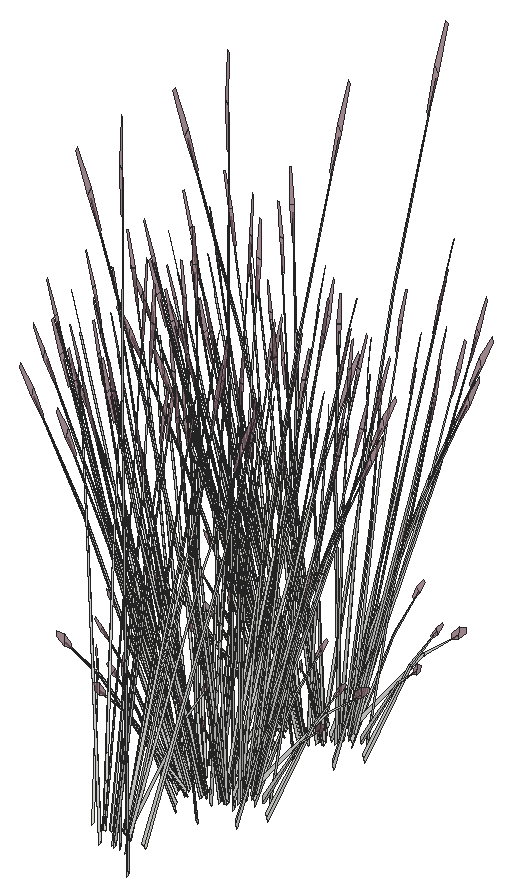
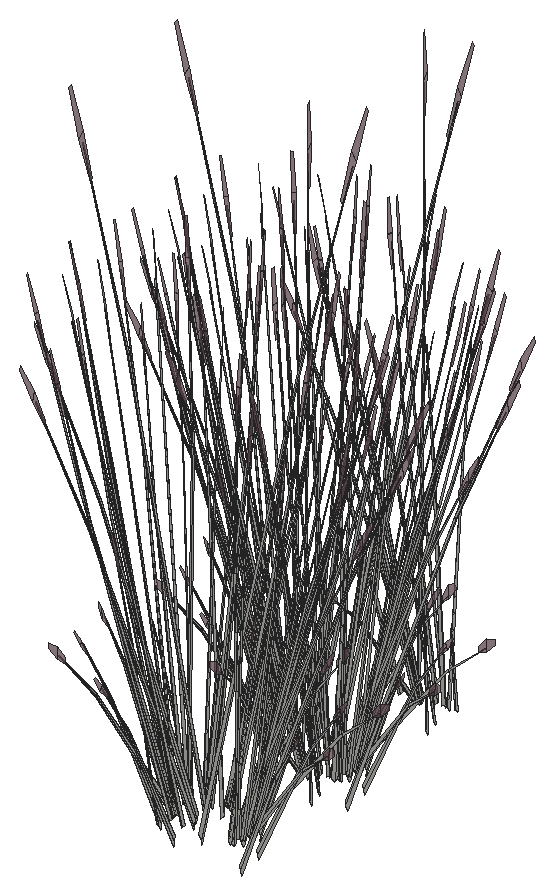
# SketchUp Ruby script. Lengths in inches.
U = 1.inch
M = Sketchup.active_model
def pt(a) = Geom::Point3d.new(a.map { |v| v * U })
def face(e, loops, mat)
  f = e.add_face(loops[0].map { |a| pt(a) })
  loops[1..].each { |l| e.add_face(l.map { |a| pt(a) }).erase! }
  f.material = f.back_material = mat if mat
  f
end
# faces: each face lists its corners as indices into pts; further lists are holes
def faces(e, pts, list, mat = nil) = list.each { |f| face(e, (f[0].is_a?(Array) ? f : [f]).map { |l| l.map { |i| pts[i] } }, mat) }
# xy, xz, yz: faces in a plane at the given z, y or x. An outline is a flat list of corners, or four numbers for a rectangle; further outlines are holes
def ring(l) = l.size == 4 ? [[l[0], l[1]], [l[2], l[1]], [l[2], l[3]], [l[0], l[3]]] : l.each_slice(2).to_a
def flat(e, list, mat, &to3) = list.each { |f| face(e, (f[0].is_a?(Array) ? f : [f]).map { |l| ring(l).map { |u, v| to3.(u, v) } }, mat) }
def xy(e, z, list, mat = nil) = flat(e, list, mat) { |x, y| [x, y, z] }
def xz(e, y, list, mat = nil) = flat(e, list, mat) { |x, z| [x, y, z] }
def yz(e, x, list, mat = nil) = flat(e, list, mat) { |y, z| [x, y, z] }
def lines(e, pts, list) = list.each { |a, b| e.add_line(pt(pts[a]), pt(pts[b])) }
# prism: a flat outline (further loops are holes) pulled along v
def prism(e, loops, v, mat = nil)
  f = face(e, loops, mat); d = Geom::Vector3d.new(v.map { |x| x * U })
  f.pushpull(f.normal.samedirection?(d) ? d.length : -d.length)
end
def box(e, o, s, mat = nil) = prism(e, [[o, [o[0] + s[0], o[1], o[2]], [o[0] + s[0], o[1] + s[1], o[2]], [o[0], o[1] + s[1], o[2]]]], [0, 0, s[2]], mat)
def at(x, y, z, deg = 0) = Geom::Transformation.translation(pt([x, y, z])) * Geom::Transformation.rotation(ORIGIN, Z_AXIS, deg.degrees)
def axes(o, x, y, z) = Geom::Transformation.new([*x, 0, *y, 0, *z, 0, *pt(o).to_a, 1])
def part(name) = M.definitions.add(name)
# library, detail: a bought-in or finely detailed component or shape, given as its bounding box
def library(name, o, s) = part(name).tap { |d| box(d.entities, o, s) }
def detail(e, o, s) = box(e.add_group.entities, o, s)
def put(e, d, t, mat = nil) = e.add_instance(d, t).tap { |i| i.material = mat if mat }
def group(e, t, mat = nil) = e.add_group.tap { |g| g.transformation = t; g.material = mat if mat }.entities
root = M.entities
M.materials.add("LightPink_Translucent").color = [144, 107, 117]
M.materials["LightPink_Translucent"].alpha = 0.75
c1 = part("blade")
p = [[2.15,0.21,22],[0,0.17,0],[0.09,0.45,0],[2.18,0.31,22],[2.29,0.31,22],[0.38,0.45,0],
  [2.48,0.24,33],[2.49,0.24,33],[2.48,0.22,33]]
faces(c1.entities,p,[[0,1,2,3],[4,5,2,3],[6,3,4,7],[8,0,3,6]])
c2 = part("seeds")
p = [[0.3,-0.1,1.38],[-0.01,-0.03,1.59],[-0.01,-0.03,0.03],[0.14,-0.07,-0.07],[0.29,-0.03,3],[0.15,0.01,3.11]]
faces(c2.entities,p,[[0,1,2,3],[1,0,4,5]],"LightPink_Translucent")
c3 = part("blade with seeds")
put(c3.entities,c1,at(0,0,0))
put(c3.entities,c2,axes([2.4,0.25,30.99],[1.5799,-0.05474,1.17369],[-0.12525,1.92788,0.29478],[-0.07173,-0.02425,1.56792]))
put(root,c3,axes([334.74,276.7,50.51],[-0.01379,-0.36791,1.24828],[0.62424,0.09537,0.52853],[-0.14764,0.20132,1.17828]))
put(root,c3,axes([334.79,278.125,52.14],[0.49824,-0.09289,-0.45151],[0.08716,0.35177,-0.34973],[0.13382,0.10081,0.86392]))
put(root,c3,axes([332.16,277.37,51.43],[0.09401,-0.13431,1.51428],[0.3944,0.27795,0.12244],[-0.17792,0.17323,0.64734]))
put(root,c3,axes([332.27,278.13,52],[-0.34164,0.20573,-0.31292],[-0.3234,-0.23491,0.40398],[-0.04921,0.11936,0.77298]))
put(root,c3,axes([331.09,278.07,52.17],[-0.01255,0.07733,1.54581],[0.35618,0.269,-0.24447],[-0.09325,0.12721,0.12397]))
put(root,c3,axes([333.25,278.3,52.45],[0.49409,-0.18193,-0.10745],[0.24281,0.32289,-0.59638],[0.06519,0.13607,0.90619]))
put(root,c3,axes([332.48,278.93,50.44],[-0.01307,-0.23234,1.01491],[0.32652,0.16572,0.74569],[-0.06422,0.11074,0.22354]))
put(root,c3,axes([332.61,278.03,52.42],[0.36145,0.26255,-0.50118],[-0.38183,0.22994,-0.3882],[-0.055,0.1334,0.95895]))
put(root,c3,axes([333.68,278.29,52.14],[0.49634,0.09796,-0.45151],[-0.17013,0.33585,-0.34973],[0.04551,0.13522,0.86392]))
put(root,c3,axes([333.96,277.59,51.43],[-0.11542,-0.12546,1.51428],[0.53333,-0.10562,0.12244],[0.12054,0.19696,0.64734]))
put(root,c3,axes([333.45,278.49,52],[-0.15222,0.30049,-0.31292],[-0.44409,-0.08764,0.40398],[0.04072,0.12098,0.77298]))
put(root,c3,axes([332.49,277.91,52.72],[-0.01314,0.36145,-0.69681],[-0.55324,-0.02428,0.08409],[-0.05838,0.15313,0.9857]))
put(root,c3,axes([333.02,277.66,51.43],[-0.01236,-0.14998,1.51428],[0.53562,0.09949,0.12244],[-0.03313,0.21373,0.64734]))
put(root,c3,axes([333.5,278.22,52.4],[0.24099,0.31773,-0.62776],[-0.49607,0.17707,0.07576],[0.05635,0.15352,0.88802]))
put(root,c3,axes([332.69,284.9375,51.43],[0.11542,0.12546,1.51428],[-0.53333,0.10562,0.12244],[-0.12054,-0.19696,0.64734]))
put(root,c3,axes([333.14,279.03,52.17],[0.064,0.06292,1.54581],[0.51651,0.02472,-0.24447],[0.05194,0.13877,0.12397]))
put(root,c3,axes([333.57,284.11,52.17],[-0.07723,-0.05479,1.54581],[-0.51538,0.03473,-0.24447],[-0.08225,-0.13104,0.12397]))
put(root,c3,axes([334.11,285.03,52.4],[-0.24099,-0.31773,-0.62776],[0.49607,-0.17707,0.07576],[-0.05635,-0.15352,0.88802]))
put(root,c3,axes([332.31,278.42,50.97],[0.01109,-0.20172,1.3638],[0.49896,0.10655,0.18846],[-0.04323,0.21498,0.64398]))
put(root,c3,axes([335.12,285.34,52.4],[0.01314,-0.36145,-0.62776],[0.55324,0.02428,0.07576],[0.05838,-0.15313,0.88802]))
put(root,c3,axes([335.89,284.78,52.17],[-0.00487,-0.07777,1.54581],[-0.41166,-0.22476,-0.24447],[0.06364,-0.13625,0.12397]))
put(root,c3,axes([334.16,284.76,52],[0.15222,-0.30049,-0.31292],[0.44409,0.08764,0.40398],[-0.04072,-0.12098,0.77298]))
put(root,c3,axes([334.5,285.16,51.43],[-0.09401,0.13431,1.51428],[-0.3944,-0.27795,0.12244],[0.17792,-0.17323,0.64734]))
put(root,c3,axes([333.93,284.97,52.14],[-0.49634,-0.09796,-0.45151],[0.17013,-0.33585,-0.34973],[-0.04551,-0.13522,0.86392]))
put(root,c3,axes([334.24,284.13,50.44],[0.06477,0.22786,1.01491],[-0.35932,-0.1262,0.74569],[0.03867,-0.11667,0.22354]))
put(root,c3,axes([335.01,285.22,52.14],[-0.36145,-0.26255,-0.45151],[0.38183,-0.22994,-0.34973],[0.055,-0.1334,0.86392]))
put(root,c3,axes([334.36,284.95,52.45],[-0.49409,0.18193,-0.10745],[-0.24281,-0.32289,-0.59638],[-0.06519,-0.13607,0.90619]))
put(root,c3,axes([335.38,285.36,52.45],[-0.55492,-0.01936,-0.10745],[0.01517,-0.36657,-0.59638],[0.03855,-0.14118,0.90619]))
put(root,c3,axes([335.35,285.125,52],[0.34164,-0.20573,-0.31292],[0.3234,0.23491,0.40398],[0.04921,-0.11936,0.77298]))
put(root,c3,axes([332.39,284.4,50.44],[0.26338,0.136,1.01491],[-0.38358,0.08175,0.74569],[-0.08207,-0.10452,0.22354]))
put(root,c3,axes([333.03,285.12,52.4],[-0.43054,-0.18887,-0.62776],[0.30598,-0.33097,0.07576],[-0.15599,-0.11277,0.88802]))
put(root,c3,axes([332.88,284.87,52],[-0.07798,-0.31474,-0.31292],[0.44579,-0.08311,0.40398],[-0.11974,-0.09019,0.77298]))
put(root,c3,axes([331.92,285.33,51.43],[0.18755,0.06732,1.51428],[-0.38813,0.28243,0.12244],[-0.24191,-0.12741,0.64734]))
put(root,c3,axes([332.83,285.13,52.14],[-0.49824,0.09289,-0.45151],[-0.08716,-0.35177,-0.34973],[-0.13382,-0.10081,0.86392]))
put(root,c3,axes([335.77,285.97,52.4],[0.26374,-0.30832,-0.62776],[0.46217,0.21911,0.07576],[0.15748,-0.11171,0.88802]))
put(root,c3,axes([335.76,285.83,52.14],[-0.12971,-0.3568,-0.45151],[0.49122,-0.06241,-0.34973],[0.14077,-0.09583,0.86392]))
put(root,c3,axes([331.88,284.71,52.17],[-0.10864,-0.00276,1.54581],[-0.34587,0.27582,-0.24447],[-0.18454,-0.05636,0.12397]))
put(root,c3,axes([335.99,286.08,52.45],[-0.46706,-0.21546,-0.10745],[0.26908,-0.31203,-0.59638],[0.13196,-0.10846,0.90619]))
put(root,c3,axes([334.06,287.26,50.9375],[0.43633,0.15757,1.33654],[-0.42745,0.33945,0.52853],[-0.19146,-0.20119,1.12046]))
put(root,c3,axes([336.36,285.12,50.44],[-0.16818,0.19891,1.01491],[-0.14456,-0.26725,0.74569],[0.1389,-0.06697,0.22354]))
put(root,c3,axes([336.12,285.86,52],[0.43951,-0.05584,-0.31292],[0.11606,0.31924,0.40398],[0.12595,-0.08575,0.77298]))
put(root,c3,axes([331.85,285.43,52],[-0.28729,-0.24465,-0.31292],[0.32804,-0.23159,0.40398],[-0.16667,-0.03524,0.77298]))
put(root,c3,axes([332.15,285.59,52.4],[-0.50473,-0.00941,-0.62776],[0.0339,-0.39618,0.07576],[-0.21383,-0.04181,0.88802]))
put(root,c3,axes([337.39,286.37,52.17],[0.07006,-0.05952,1.54581],[-0.08968,-0.3651,-0.24447],[0.1758,-0.06922,0.12397]))
put(root,c3,axes([331.98,285.67,52.14],[-0.36663,0.25884,-0.45151],[-0.32109,-0.27343,-0.34973],[-0.18628,-0.03938,0.86392]))
put(root,c3,axes([331.16,286.01,50.44],[0.32236,-0.02796,1.01491],[-0.20448,0.24636,0.74569],[-0.1593,-0.03696,0.22354]))
put(root,c3,axes([332.18,285.4,52.45],[-0.02704,0.39739,-0.10745],[-0.51189,-0.01086,-0.59638],[-0.19715,-0.0276,0.90619]))
put(root,c3,axes([336.01,286.92,52.45],[-0.25405,-0.35383,-0.10745],[0.45089,-0.17388,-0.59638],[0.19001,-0.04668,0.90619]))
put(root,c3,axes([335.98,286.62,52.14],[0.13679,-0.35544,-0.45151],[0.46898,0.12183,-0.34973],[0.18882,-0.03259,0.86392]))
put(root,c3,axes([331.52,285.95,51.43],[0.20943,-0.00885,1.51428],[-0.13893,0.38357,0.12244],[-0.29846,-0.02372,0.64734]))
put(root,c3,axes([335.9,286.75,52.4],[0.44368,-0.17257,-0.62776],[0.24726,0.35524,0.07576],[0.21437,-0.04035,0.88802]))
put(root,c3,axes([336.27,286.78,52],[0.41962,0.10901,-0.31292],[-0.12239,0.31802,0.40398],[0.16894,-0.02916,0.77298]))
put(root,c3,axes([331.34,286.28,52],[-0.41962,-0.10901,-0.31292],[0.12239,-0.31802,0.40398],[-0.16894,0.02916,0.77298]))
put(root,c3,axes([335.13,286.39,51.43],[-0.20943,0.00885,1.51428],[0.13893,-0.38357,0.12244],[0.29846,0.02372,0.64734]))
put(root,c3,axes([332.62,286.22,50.95],[0.14352,-0.05653,1.56454],[0.04949,0.39467,0.12244],[-0.31087,0.05237,0.55918]))
put(root,c3,axes([337.16,286.85,50.44],[-0.31197,0.06451,1.01491],[0.14684,-0.26661,0.74569],[0.1655,0.01824,0.22354]))
put(root,c3,axes([331.08,286.49,52.17],[-0.08245,0.05073,1.54581],[0.00701,0.37067,-0.24447],[-0.18899,0.0482,0.12397]))
put(root,c3,axes([331.63,286.4375,52.14],[-0.13679,0.35544,-0.45151],[-0.46898,-0.12183,-0.34973],[-0.18882,0.03259,0.86392]))
put(root,c3,axes([331.61,286.13,52.45],[0.25405,0.35383,-0.10745],[-0.45089,0.17388,-0.59638],[-0.19001,0.04668,0.90619]))
put(root,c3,axes([336.62,287.67,51.47],[-0.09664,-0.32847,-0.03085],[0.45676,-0.07551,-0.13989],[0.09538,0.02082,0.4614]))
put(root,c3,axes([335.4375,287.66,52.45],[0.02704,-0.39739,-0.10745],[0.51189,0.01086,-0.59638],[0.19715,0.0276,0.90619]))
put(root,c3,axes([335.88,287.42,52.17],[0.10831,-0.00661,1.54581],[0.29709,-0.30358,-0.24447],[0.19266,0.04007,0.12397]))
put(root,c3,axes([331.61,286.62,51.43],[0.17519,-0.08265,1.51428],[0.14749,0.38193,0.12244],[-0.27504,0.08632,0.64734]))
put(root,c3,axes([335.46,287.47,52.4],[0.50473,0.00941,-0.62776],[-0.0339,0.39618,0.07576],[0.21383,0.04181,0.88802]))
put(root,c3,axes([330.7,287.96,50.44],[0.21042,-0.1771,1.01491],[0.08303,0.28036,0.74569],[-0.15207,0.0502,0.22354]))
put(root,c3,axes([335.77,287.63,52],[0.28729,0.24465,-0.31292],[-0.32804,0.23159,0.40398],[0.16667,0.03524,0.77298]))
put(root,c3,axes([331.49,287.19,52],[-0.43951,0.05584,-0.31292],[-0.11606,-0.31924,0.40398],[-0.12595,0.08575,0.77298]))
put(root,c3,axes([334.73,287,51.43],[-0.18755,-0.06732,1.51428],[0.38813,-0.28243,0.12244],[0.24191,0.12741,0.64734]))
put(root,c3,axes([334.77,286.12,51.95],[-0.4363,-0.20303,1.22187],[0.46069,-0.31611,0.5272],[0.14077,0.1905,1.18105]))
put(root,c3,axes([331.625,286.97,52.45],[0.46706,0.21546,-0.10745],[-0.26908,0.31203,-0.59638],[-0.13196,0.10846,0.90619]))
put(root,c3,axes([335.43,287.77,50.44],[-0.28429,-0.11236,1.01491],[0.36709,-0.11416,0.74569],[0.09901,0.0967,0.22354]))
put(root,c3,axes([334.43,288.09,52.45],[0.30087,-0.33447,-0.10745],[0.43572,0.19269,-0.59638],[0.15146,0.0945,0.90619]))
put(root,c3,axes([332.25,286.88,51.43],[0.12611,-0.12006,1.51428],[0.31843,0.32408,0.12244],[-0.2184,0.14759,0.64734]))
put(root,c3,axes([331.86,287.23,52.14],[0.12971,0.3568,-0.45151],[-0.49122,0.06241,-0.34973],[-0.14077,0.09583,0.86392]))
put(root,c3,axes([334.74,286.51,50.51],[-0.01379,-0.36791,1.24828],[0.62424,0.09537,0.52853],[-0.14764,0.20132,1.17828]))
put(root,c3,axes([334.79,287.93,52.14],[0.49824,-0.09289,-0.45151],[0.08716,0.35177,-0.34973],[0.13382,0.10081,0.86392]))
put(root,c3,axes([332.16,287.17,51.43],[0.09401,-0.13431,1.51428],[0.3944,0.27795,0.12244],[-0.17792,0.17323,0.64734]))
put(root,c3,axes([332.27,287.93,52],[-0.34164,0.20573,-0.31292],[-0.3234,-0.23491,0.40398],[-0.04921,0.11936,0.77298]))
put(root,c3,axes([331.09,287.87,52.17],[-0.01255,0.07733,1.54581],[0.35618,0.269,-0.24447],[-0.09325,0.12721,0.12397]))
put(root,c3,axes([333.25,288.1,52.45],[0.49409,-0.18193,-0.10745],[0.24281,0.32289,-0.59638],[0.06519,0.13607,0.90619]))
put(root,c3,axes([332.48,288.73,50.44],[-0.01307,-0.23234,1.01491],[0.32652,0.16572,0.74569],[-0.06422,0.11074,0.22354]))
put(root,c3,axes([332.69,293.92,51.43],[0.11542,0.12546,1.51428],[-0.53333,0.10562,0.12244],[-0.12054,-0.19696,0.64734]))
put(root,c3,axes([333.57,293.08,52.17],[-0.07723,-0.05479,1.54581],[-0.51538,0.03473,-0.24447],[-0.08225,-0.13104,0.12397]))
put(root,c3,axes([332.61,287.83,52.42],[0.36145,0.26255,-0.50118],[-0.38183,0.22994,-0.3882],[-0.055,0.1334,0.95895]))
put(root,c3,axes([334.11,294.01,52.4],[-0.24099,-0.31773,-0.62776],[0.49607,-0.17707,0.07576],[-0.05635,-0.15352,0.88802]))
put(root,c3,axes([333.68,288.09,52.14],[0.49634,0.09796,-0.45151],[-0.17013,0.33585,-0.34973],[0.04551,0.13522,0.86392]))
put(root,c3,axes([333.96,287.4,51.43],[-0.11542,-0.12546,1.51428],[0.53333,-0.10562,0.12244],[0.12054,0.19696,0.64734]))
put(root,c3,axes([333.45,288.29,52],[-0.15222,0.30049,-0.31292],[-0.44409,-0.08764,0.40398],[0.04072,0.12098,0.77298]))
put(root,c3,axes([332.49,287.71,52.72],[-0.01314,0.36145,-0.69681],[-0.55324,-0.02428,0.08409],[-0.05838,0.15313,0.9857]))
put(root,c3,axes([335.12,294.32,52.4],[0.01314,-0.36145,-0.62776],[0.55324,0.02428,0.07576],[0.05838,-0.15313,0.88802]))
put(root,c3,axes([335.89,293.76,52.17],[-0.00487,-0.07777,1.54581],[-0.41166,-0.22476,-0.24447],[0.06364,-0.13625,0.12397]))
put(root,c3,axes([333.02,287.46,51.43],[-0.01236,-0.14998,1.51428],[0.53562,0.09949,0.12244],[-0.03313,0.21373,0.64734]))
put(root,c3,axes([334.16,293.74,52],[0.15222,-0.30049,-0.31292],[0.44409,0.08764,0.40398],[-0.04072,-0.12098,0.77298]))
put(root,c3,axes([334.5,294.14,51.43],[-0.09401,0.13431,1.51428],[-0.3944,-0.27795,0.12244],[0.17792,-0.17323,0.64734]))
put(root,c3,axes([333.93,293.95,52.14],[-0.49634,-0.09796,-0.45151],[0.17013,-0.33585,-0.34973],[-0.04551,-0.13522,0.86392]))
put(root,c3,axes([334.24,293.1,50.44],[0.06477,0.22786,1.01491],[-0.35932,-0.1262,0.74569],[0.03867,-0.11667,0.22354]))
put(root,c3,axes([333.5,288.02,52.4],[0.24099,0.31773,-0.62776],[-0.49607,0.17707,0.07576],[0.05635,0.15352,0.88802]))
put(root,c3,axes([335.01,294.2,52.14],[-0.36145,-0.26255,-0.45151],[0.38183,-0.22994,-0.34973],[0.055,-0.1334,0.86392]))
put(root,c3,axes([333.14,288.83,52.17],[0.064,0.06292,1.54581],[0.51651,0.02472,-0.24447],[0.05194,0.13877,0.12397]))
put(root,c3,axes([334.36,293.93,52.45],[-0.49409,0.18193,-0.10745],[-0.24281,-0.32289,-0.59638],[-0.06519,-0.13607,0.90619]))
put(root,c3,axes([335.38,294.34,52.45],[-0.55492,-0.01936,-0.10745],[0.01517,-0.36657,-0.59638],[0.03855,-0.14118,0.90619]))
put(root,c3,axes([335.35,294.1,52],[0.34164,-0.20573,-0.31292],[0.3234,0.23491,0.40398],[0.04921,-0.11936,0.77298]))
put(root,c3,axes([332.39,293.38,50.44],[0.26338,0.136,1.01491],[-0.38358,0.08175,0.74569],[-0.08207,-0.10452,0.22354]))
put(root,c3,axes([333.03,294.1,52.4],[-0.43054,-0.18887,-0.62776],[0.30598,-0.33097,0.07576],[-0.15599,-0.11277,0.88802]))
put(root,c3,axes([332.88,293.85,52],[-0.07798,-0.31474,-0.31292],[0.44579,-0.08311,0.40398],[-0.11974,-0.09019,0.77298]))
put(root,c3,axes([332.31,288.22,50.97],[0.01109,-0.20172,1.3638],[0.49896,0.10655,0.18846],[-0.04323,0.21498,0.64398]))
put(root,c3,axes([331.92,294.31,51.43],[0.18755,0.06732,1.51428],[-0.38813,0.28243,0.12244],[-0.24191,-0.12741,0.64734]))
put(root,c3,axes([332.83,294.11,52.14],[-0.49824,0.09289,-0.45151],[-0.08716,-0.35177,-0.34973],[-0.13382,-0.10081,0.86392]))
put(root,c3,axes([335.77,294.95,52.4],[0.26374,-0.30832,-0.62776],[0.46217,0.21911,0.07576],[0.15748,-0.11171,0.88802]))
put(root,c3,axes([335.76,294.8,52.14],[-0.12971,-0.3568,-0.45151],[0.49122,-0.06241,-0.34973],[0.14077,-0.09583,0.86392]))
put(root,c3,axes([331.88,293.6875,52.17],[-0.10864,-0.00276,1.54581],[-0.34587,0.27582,-0.24447],[-0.18454,-0.05636,0.12397]))
put(root,c3,axes([335.99,295.06,52.45],[-0.46706,-0.21546,-0.10745],[0.26908,-0.31203,-0.59638],[0.13196,-0.10846,0.90619]))
put(root,c3,axes([334.06,296.24,50.9375],[0.43633,0.15757,1.33654],[-0.42745,0.33945,0.52853],[-0.19146,-0.20119,1.12046]))
put(root,c3,axes([336.36,294.09,50.44],[-0.16818,0.19891,1.01491],[-0.14456,-0.26725,0.74569],[0.1389,-0.06697,0.22354]))
put(root,c3,axes([336.12,294.84,52],[0.43951,-0.05584,-0.31292],[0.11606,0.31924,0.40398],[0.12595,-0.08575,0.77298]))
put(root,c3,axes([331.85,294.4,52],[-0.28729,-0.24465,-0.31292],[0.32804,-0.23159,0.40398],[-0.16667,-0.03524,0.77298]))
put(root,c3,axes([332.15,294.57,52.4],[-0.50473,-0.00941,-0.62776],[0.0339,-0.39618,0.07576],[-0.21383,-0.04181,0.88802]))
put(root,c3,axes([337.39,295.35,52.17],[0.07006,-0.05952,1.54581],[-0.08968,-0.3651,-0.24447],[0.1758,-0.06922,0.12397]))
put(root,c3,axes([331.98,294.65,52.14],[-0.36663,0.25884,-0.45151],[-0.32109,-0.27343,-0.34973],[-0.18628,-0.03938,0.86392]))
put(root,c3,axes([331.16,294.99,50.44],[0.32236,-0.02796,1.01491],[-0.20448,0.24636,0.74569],[-0.1593,-0.03696,0.22354]))
put(root,c3,axes([332.18,294.375,52.45],[-0.02704,0.39739,-0.10745],[-0.51189,-0.01086,-0.59638],[-0.19715,-0.0276,0.90619]))
put(root,c3,axes([336.01,295.9,52.45],[-0.25405,-0.35383,-0.10745],[0.45089,-0.17388,-0.59638],[0.19001,-0.04668,0.90619]))
put(root,c3,axes([335.98,295.6,52.14],[0.13679,-0.35544,-0.45151],[0.46898,0.12183,-0.34973],[0.18882,-0.03259,0.86392]))
put(root,c3,axes([331.52,294.92,51.43],[0.20943,-0.00885,1.51428],[-0.13893,0.38357,0.12244],[-0.29846,-0.02372,0.64734]))
put(root,c3,axes([335.9,295.73,52.4],[0.44368,-0.17257,-0.62776],[0.24726,0.35524,0.07576],[0.21437,-0.04035,0.88802]))
put(root,c3,axes([336.27,295.76,52],[0.41962,0.10901,-0.31292],[-0.12239,0.31802,0.40398],[0.16894,-0.02916,0.77298]))
put(root,c3,axes([331.34,295.25,52],[-0.41962,-0.10901,-0.31292],[0.12239,-0.31802,0.40398],[-0.16894,0.02916,0.77298]))
put(root,c3,axes([335.13,295.37,51.43],[-0.20943,0.00885,1.51428],[0.13893,-0.38357,0.12244],[0.29846,0.02372,0.64734]))
put(root,c3,axes([332.62,295.2,50.95],[0.14352,-0.05653,1.56454],[0.04949,0.39467,0.12244],[-0.31087,0.05237,0.55918]))
put(root,c3,axes([337.16,295.82,50.44],[-0.31197,0.06451,1.01491],[0.14684,-0.26661,0.74569],[0.1655,0.01824,0.22354]))
put(root,c3,axes([331.08,295.46,52.17],[-0.08245,0.05073,1.54581],[0.00701,0.37067,-0.24447],[-0.18899,0.0482,0.12397]))
put(root,c3,axes([331.63,295.41,52.14],[-0.13679,0.35544,-0.45151],[-0.46898,-0.12183,-0.34973],[-0.18882,0.03259,0.86392]))
put(root,c3,axes([331.61,295.11,52.45],[0.25405,0.35383,-0.10745],[-0.45089,0.17388,-0.59638],[-0.19001,0.04668,0.90619]))
put(root,c3,axes([336.62,296.65,51.47],[-0.09664,-0.32847,-0.03085],[0.45676,-0.07551,-0.13989],[0.09538,0.02082,0.4614]))
put(root,c3,axes([335.4375,296.64,52.45],[0.02704,-0.39739,-0.10745],[0.51189,0.01086,-0.59638],[0.19715,0.0276,0.90619]))
put(root,c3,axes([335.88,296.4,52.17],[0.10831,-0.00661,1.54581],[0.29709,-0.30358,-0.24447],[0.19266,0.04007,0.12397]))
put(root,c3,axes([331.61,295.6,51.43],[0.17519,-0.08265,1.51428],[0.14749,0.38193,0.12244],[-0.27504,0.08632,0.64734]))
put(root,c3,axes([335.46,296.44,52.4],[0.50473,0.00941,-0.62776],[-0.0339,0.39618,0.07576],[0.21383,0.04181,0.88802]))
put(root,c3,axes([330.7,296.93,50.44],[0.21042,-0.1771,1.01491],[0.08303,0.28036,0.74569],[-0.15207,0.0502,0.22354]))
put(root,c3,axes([335.77,296.61,52],[0.28729,0.24465,-0.31292],[-0.32804,0.23159,0.40398],[0.16667,0.03524,0.77298]))
put(root,c3,axes([331.49,296.17,52],[-0.43951,0.05584,-0.31292],[-0.11606,-0.31924,0.40398],[-0.12595,0.08575,0.77298]))
put(root,c3,axes([334.73,295.98,51.43],[-0.18755,-0.06732,1.51428],[0.38813,-0.28243,0.12244],[0.24191,0.12741,0.64734]))
put(root,c3,axes([334.77,295.09,51.95],[-0.4363,-0.20303,1.22187],[0.46069,-0.31611,0.5272],[0.14077,0.1905,1.18105]))
put(root,c3,axes([331.625,295.95,52.45],[0.46706,0.21546,-0.10745],[-0.26908,0.31203,-0.59638],[-0.13196,0.10846,0.90619]))
put(root,c3,axes([335.43,296.75,50.44],[-0.28429,-0.11236,1.01491],[0.36709,-0.11416,0.74569],[0.09901,0.0967,0.22354]))
put(root,c3,axes([334.43,297.07,52.45],[0.30087,-0.33447,-0.10745],[0.43572,0.19269,-0.59638],[0.15146,0.0945,0.90619]))
put(root,c3,axes([332.25,295.85,51.43],[0.12611,-0.12006,1.51428],[0.31843,0.32408,0.12244],[-0.2184,0.14759,0.64734]))
put(root,c3,axes([331.86,296.21,52.14],[0.12971,0.3568,-0.45151],[-0.49122,0.06241,-0.34973],[-0.14077,0.09583,0.86392]))
